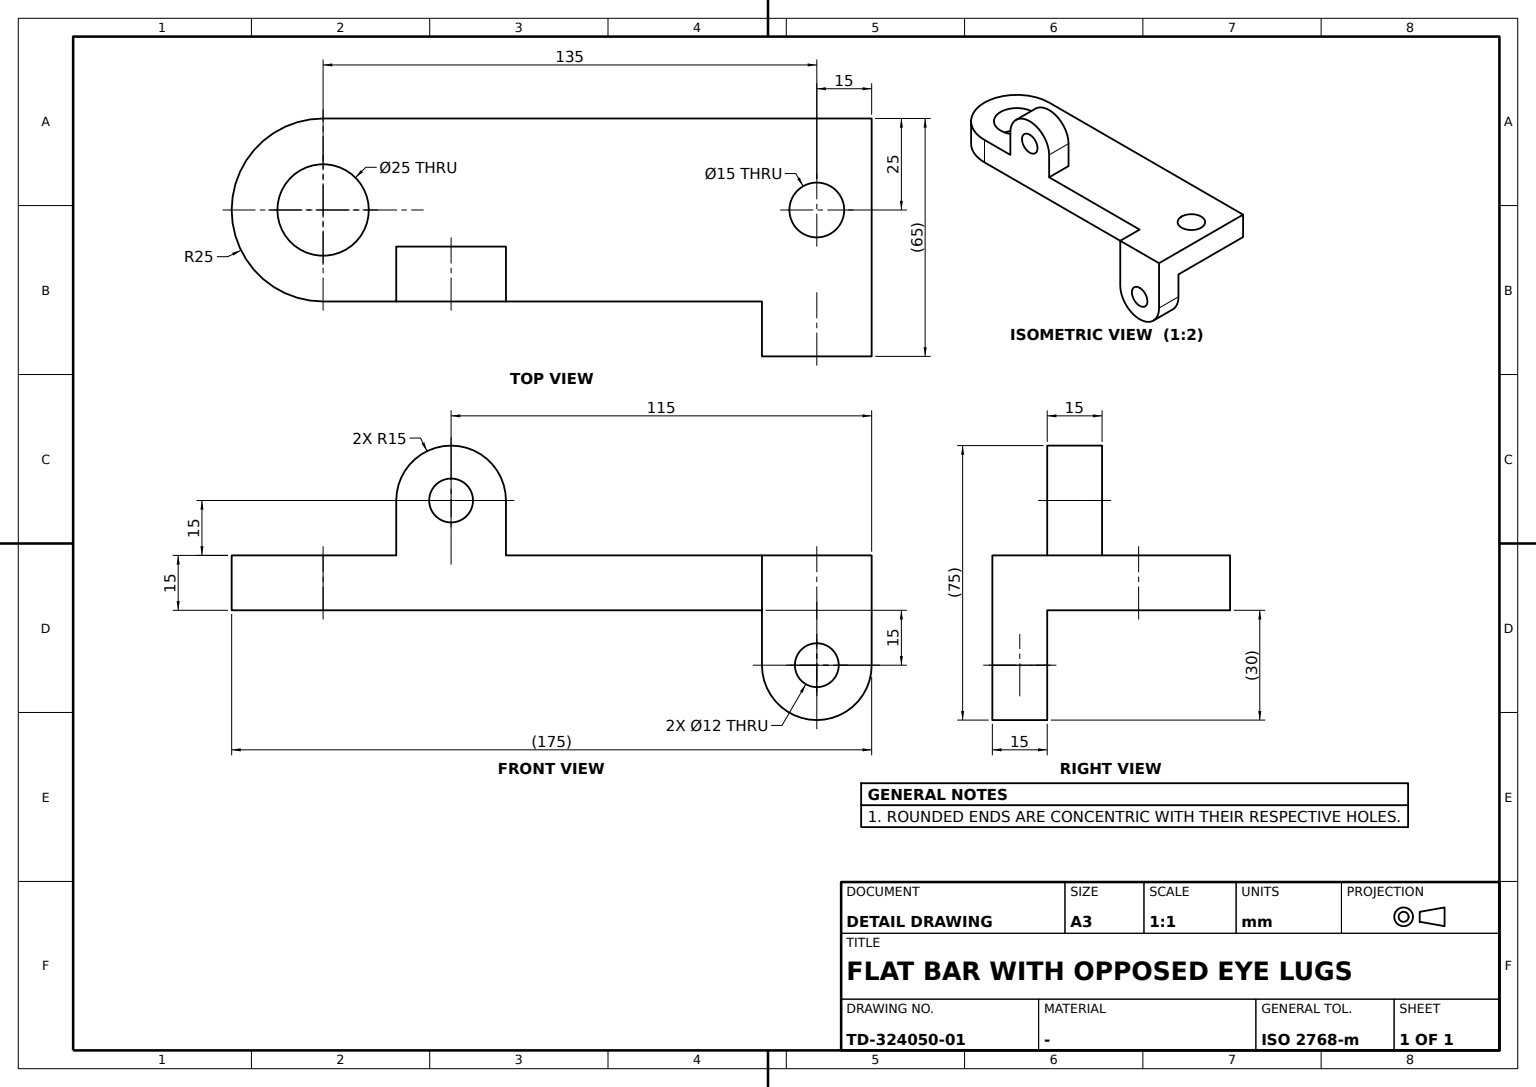
ISO-10303-21;
HEADER;
FILE_DESCRIPTION((''),'2;1');
FILE_NAME('','',(''),(''),'','','');
FILE_SCHEMA(('AUTOMOTIVE_DESIGN'));
ENDSEC;
DATA;
#1=APPLICATION_CONTEXT('');
#2=PRODUCT_CONTEXT('',#1,'mechanical');
#3=PRODUCT('','','',(#2));
#4=PRODUCT_DEFINITION_FORMATION('','',#3);
#5=PRODUCT_DEFINITION_CONTEXT('',#1,'design');
#6=PRODUCT_DEFINITION('','',#4,#5);
#7=PRODUCT_DEFINITION_SHAPE('','',#6);
#8=(LENGTH_UNIT()NAMED_UNIT(*)SI_UNIT(.MILLI.,.METRE.));
#9=(NAMED_UNIT(*)PLANE_ANGLE_UNIT()SI_UNIT($,.RADIAN.));
#10=(NAMED_UNIT(*)SI_UNIT($,.STERADIAN.)SOLID_ANGLE_UNIT());
#11=UNCERTAINTY_MEASURE_WITH_UNIT(LENGTH_MEASURE(0.005),#8,'distance_accuracy_value','');
#12=(GEOMETRIC_REPRESENTATION_CONTEXT(3)GLOBAL_UNCERTAINTY_ASSIGNED_CONTEXT((#11))GLOBAL_UNIT_ASSIGNED_CONTEXT((#8,#9,#10))REPRESENTATION_CONTEXT('',''));
#13=CARTESIAN_POINT('',(127.5,0.,-15.));
#14=VERTEX_POINT('',#13);
#15=CARTESIAN_POINT('',(127.5,0.,0.));
#16=VERTEX_POINT('',#15);
#17=DIRECTION('',(0.,0.,-1.));
#18=VECTOR('',#17,1000.);
#19=LINE('',#15,#18);
#20=EDGE_CURVE('',#14,#16,#19,.F.);
#21=ORIENTED_EDGE('',*,*,#20,.F.);
#22=CARTESIAN_POINT('',(142.5,0.,-15.));
#23=VERTEX_POINT('',#22);
#24=CARTESIAN_POINT('',(135.,0.,-15.));
#25=DIRECTION('',(0.,0.,1.));
#26=DIRECTION('',(1.,0.,0.));
#27=AXIS2_PLACEMENT_3D('',#24,#25,#26);
#28=CIRCLE('',#27,7.5);
#29=EDGE_CURVE('',#23,#14,#28,.T.);
#30=ORIENTED_EDGE('',*,*,#29,.F.);
#31=CARTESIAN_POINT('',(142.5,0.,0.));
#32=VERTEX_POINT('',#31);
#33=LINE('',#31,#18);
#34=EDGE_CURVE('',#32,#23,#33,.T.);
#35=ORIENTED_EDGE('',*,*,#34,.F.);
#36=CARTESIAN_POINT('',(135.,0.,0.));
#37=AXIS2_PLACEMENT_3D('',#36,#25,#26);
#38=CIRCLE('',#37,7.5);
#39=EDGE_CURVE('',#32,#16,#38,.T.);
#40=ORIENTED_EDGE('',*,*,#39,.T.);
#41=EDGE_LOOP('',(#21,#30,#35,#40));
#42=FACE_BOUND('',#41,.T.);
#43=DIRECTION('',(-1.,0.,0.));
#44=AXIS2_PLACEMENT_3D('',#36,#17,#43);
#45=CYLINDRICAL_SURFACE('',#44,7.5);
#46=ADVANCED_FACE('',(#42),#45,.F.);
#47=CARTESIAN_POINT('',(35.,-25.,30.));
#48=VERTEX_POINT('',#47);
#49=CARTESIAN_POINT('',(35.,-10.,30.));
#50=VERTEX_POINT('',#49);
#51=DIRECTION('',(0.,1.,0.));
#52=VECTOR('',#51,1000.);
#53=LINE('',#47,#52);
#54=EDGE_CURVE('',#48,#50,#53,.T.);
#55=ORIENTED_EDGE('',*,*,#54,.T.);
#56=CARTESIAN_POINT('',(20.,-10.,15.));
#57=VERTEX_POINT('',#56);
#58=CARTESIAN_POINT('',(35.,-10.,15.));
#59=DIRECTION('',(0.,-1.,0.));
#60=AXIS2_PLACEMENT_3D('',#58,#59,#26);
#61=CIRCLE('',#60,15.);
#62=EDGE_CURVE('',#50,#57,#61,.T.);
#63=ORIENTED_EDGE('',*,*,#62,.T.);
#64=CARTESIAN_POINT('',(20.,-25.,15.));
#65=VERTEX_POINT('',#64);
#66=LINE('',#64,#52);
#67=EDGE_CURVE('',#65,#57,#66,.T.);
#68=ORIENTED_EDGE('',*,*,#67,.F.);
#69=CARTESIAN_POINT('',(35.,-25.,15.));
#70=AXIS2_PLACEMENT_3D('',#69,#59,#26);
#71=CIRCLE('',#70,15.);
#72=EDGE_CURVE('',#48,#65,#71,.T.);
#73=ORIENTED_EDGE('',*,*,#72,.F.);
#74=EDGE_LOOP('',(#55,#63,#68,#73));
#75=FACE_BOUND('',#74,.T.);
#76=AXIS2_PLACEMENT_3D('',#69,#51,#25);
#77=CYLINDRICAL_SURFACE('',#76,15.);
#78=ADVANCED_FACE('',(#75),#77,.T.);
#79=CARTESIAN_POINT('',(50.,-25.,15.));
#80=VERTEX_POINT('',#79);
#81=EDGE_CURVE('',#80,#48,#71,.T.);
#82=ORIENTED_EDGE('',*,*,#81,.F.);
#83=CARTESIAN_POINT('',(50.,-10.,15.));
#84=VERTEX_POINT('',#83);
#85=LINE('',#79,#52);
#86=EDGE_CURVE('',#80,#84,#85,.T.);
#87=ORIENTED_EDGE('',*,*,#86,.T.);
#88=EDGE_CURVE('',#84,#50,#61,.T.);
#89=ORIENTED_EDGE('',*,*,#88,.T.);
#90=ORIENTED_EDGE('',*,*,#54,.F.);
#91=EDGE_LOOP('',(#82,#87,#89,#90));
#92=FACE_BOUND('',#91,.T.);
#93=ADVANCED_FACE('',(#92),#77,.T.);
#94=CARTESIAN_POINT('',(135.,-25.,-36.));
#95=VERTEX_POINT('',#94);
#96=CARTESIAN_POINT('',(135.,-25.,-24.));
#97=VERTEX_POINT('',#96);
#98=CARTESIAN_POINT('',(135.,-25.,-30.));
#99=AXIS2_PLACEMENT_3D('',#98,#59,#26);
#100=CIRCLE('',#99,6.);
#101=EDGE_CURVE('',#95,#97,#100,.T.);
#102=ORIENTED_EDGE('',*,*,#101,.T.);
#103=EDGE_CURVE('',#97,#95,#100,.T.);
#104=ORIENTED_EDGE('',*,*,#103,.T.);
#105=EDGE_LOOP('',(#102,#104));
#106=FACE_BOUND('',#105,.T.);
#107=CARTESIAN_POINT('',(120.,-25.,-15.));
#108=VERTEX_POINT('',#107);
#109=CARTESIAN_POINT('',(150.,-25.,-15.));
#110=VERTEX_POINT('',#109);
#111=CARTESIAN_POINT('',(0.,-25.,-15.));
#112=VECTOR('',#26,1000.);
#113=LINE('',#111,#112);
#114=EDGE_CURVE('',#108,#110,#113,.T.);
#115=ORIENTED_EDGE('',*,*,#114,.T.);
#116=CARTESIAN_POINT('',(150.,-25.,-30.));
#117=VERTEX_POINT('',#116);
#118=VECTOR('',#25,1000.);
#119=LINE('',#116,#118);
#120=EDGE_CURVE('',#117,#110,#119,.T.);
#121=ORIENTED_EDGE('',*,*,#120,.F.);
#122=CARTESIAN_POINT('',(135.,-25.,-45.));
#123=VERTEX_POINT('',#122);
#124=CIRCLE('',#99,15.);
#125=EDGE_CURVE('',#123,#117,#124,.T.);
#126=ORIENTED_EDGE('',*,*,#125,.F.);
#127=CARTESIAN_POINT('',(120.,-25.,-30.));
#128=VERTEX_POINT('',#127);
#129=EDGE_CURVE('',#128,#123,#124,.T.);
#130=ORIENTED_EDGE('',*,*,#129,.F.);
#131=CARTESIAN_POINT('',(120.,-25.,0.));
#132=LINE('',#131,#18);
#133=EDGE_CURVE('',#108,#128,#132,.T.);
#134=ORIENTED_EDGE('',*,*,#133,.F.);
#135=EDGE_LOOP('',(#115,#121,#126,#130,#134));
#136=FACE_BOUND('',#135,.T.);
#137=AXIS2_PLACEMENT_3D('',#98,#59,#17);
#138=PLANE('',#137);
#139=ADVANCED_FACE('',(#106,#136),#138,.F.);
#140=CARTESIAN_POINT('',(135.,-40.,-24.));
#141=VERTEX_POINT('',#140);
#142=VECTOR('',#59,1000.);
#143=LINE('',#96,#142);
#144=EDGE_CURVE('',#141,#97,#143,.F.);
#145=ORIENTED_EDGE('',*,*,#144,.T.);
#146=ORIENTED_EDGE('',*,*,#101,.F.);
#147=CARTESIAN_POINT('',(135.,-40.,-36.));
#148=VERTEX_POINT('',#147);
#149=LINE('',#94,#142);
#150=EDGE_CURVE('',#95,#148,#149,.T.);
#151=ORIENTED_EDGE('',*,*,#150,.T.);
#152=CARTESIAN_POINT('',(135.,-40.,-30.));
#153=AXIS2_PLACEMENT_3D('',#152,#59,#26);
#154=CIRCLE('',#153,6.);
#155=EDGE_CURVE('',#148,#141,#154,.T.);
#156=ORIENTED_EDGE('',*,*,#155,.T.);
#157=EDGE_LOOP('',(#145,#146,#151,#156));
#158=FACE_BOUND('',#157,.T.);
#159=CYLINDRICAL_SURFACE('',#137,6.);
#160=ADVANCED_FACE('',(#158),#159,.F.);
#161=ORIENTED_EDGE('',*,*,#86,.F.);
#162=CARTESIAN_POINT('',(50.,-25.,0.));
#163=VERTEX_POINT('',#162);
#164=LINE('',#162,#118);
#165=EDGE_CURVE('',#163,#80,#164,.T.);
#166=ORIENTED_EDGE('',*,*,#165,.F.);
#167=CARTESIAN_POINT('',(50.,-10.,0.));
#168=VERTEX_POINT('',#167);
#169=LINE('',#162,#52);
#170=EDGE_CURVE('',#163,#168,#169,.T.);
#171=ORIENTED_EDGE('',*,*,#170,.T.);
#172=LINE('',#167,#118);
#173=EDGE_CURVE('',#168,#84,#172,.T.);
#174=ORIENTED_EDGE('',*,*,#173,.T.);
#175=EDGE_LOOP('',(#161,#166,#171,#174));
#176=FACE_BOUND('',#175,.T.);
#177=AXIS2_PLACEMENT_3D('',#162,#43,#25);
#178=PLANE('',#177);
#179=ADVANCED_FACE('',(#176),#178,.F.);
#180=EDGE_CURVE('',#16,#32,#38,.T.);
#181=ORIENTED_EDGE('',*,*,#180,.T.);
#182=ORIENTED_EDGE('',*,*,#34,.T.);
#183=EDGE_CURVE('',#14,#23,#28,.T.);
#184=ORIENTED_EDGE('',*,*,#183,.F.);
#185=ORIENTED_EDGE('',*,*,#20,.T.);
#186=EDGE_LOOP('',(#181,#182,#184,#185));
#187=FACE_BOUND('',#186,.T.);
#188=ADVANCED_FACE('',(#187),#45,.F.);
#189=CARTESIAN_POINT('',(150.,25.,-15.));
#190=VERTEX_POINT('',#189);
#191=LINE('',#109,#52);
#192=EDGE_CURVE('',#110,#190,#191,.T.);
#193=ORIENTED_EDGE('',*,*,#192,.T.);
#194=CARTESIAN_POINT('',(150.,25.,0.));
#195=VERTEX_POINT('',#194);
#196=LINE('',#194,#18);
#197=EDGE_CURVE('',#195,#190,#196,.T.);
#198=ORIENTED_EDGE('',*,*,#197,.F.);
#199=CARTESIAN_POINT('',(150.,-40.,0.));
#200=VERTEX_POINT('',#199);
#201=CARTESIAN_POINT('',(150.,-25.,0.));
#202=LINE('',#201,#52);
#203=EDGE_CURVE('',#200,#195,#202,.T.);
#204=ORIENTED_EDGE('',*,*,#203,.F.);
#205=CARTESIAN_POINT('',(150.,-40.,-30.));
#206=VERTEX_POINT('',#205);
#207=LINE('',#205,#118);
#208=EDGE_CURVE('',#206,#200,#207,.T.);
#209=ORIENTED_EDGE('',*,*,#208,.F.);
#210=LINE('',#116,#142);
#211=EDGE_CURVE('',#117,#206,#210,.T.);
#212=ORIENTED_EDGE('',*,*,#211,.F.);
#213=ORIENTED_EDGE('',*,*,#120,.T.);
#214=EDGE_LOOP('',(#193,#198,#204,#209,#212,#213));
#215=FACE_BOUND('',#214,.T.);
#216=AXIS2_PLACEMENT_3D('',#201,#43,#25);
#217=PLANE('',#216);
#218=ADVANCED_FACE('',(#215),#217,.F.);
#219=CARTESIAN_POINT('',(-25.,0.,-15.));
#220=VERTEX_POINT('',#219);
#221=VERTEX_POINT('',#111);
#222=CARTESIAN_POINT('',(0.,0.,-15.));
#223=AXIS2_PLACEMENT_3D('',#222,#25,#26);
#224=CIRCLE('',#223,25.);
#225=EDGE_CURVE('',#220,#221,#224,.T.);
#226=ORIENTED_EDGE('',*,*,#225,.T.);
#227=CARTESIAN_POINT('',(0.,-25.,0.));
#228=VERTEX_POINT('',#227);
#229=LINE('',#227,#18);
#230=EDGE_CURVE('',#228,#221,#229,.T.);
#231=ORIENTED_EDGE('',*,*,#230,.F.);
#232=CARTESIAN_POINT('',(-25.,0.,0.));
#233=VERTEX_POINT('',#232);
#234=CARTESIAN_POINT('',(0.,0.,0.));
#235=AXIS2_PLACEMENT_3D('',#234,#25,#26);
#236=CIRCLE('',#235,25.);
#237=EDGE_CURVE('',#233,#228,#236,.T.);
#238=ORIENTED_EDGE('',*,*,#237,.F.);
#239=LINE('',#232,#18);
#240=EDGE_CURVE('',#233,#220,#239,.T.);
#241=ORIENTED_EDGE('',*,*,#240,.T.);
#242=EDGE_LOOP('',(#226,#231,#238,#241));
#243=FACE_BOUND('',#242,.T.);
#244=AXIS2_PLACEMENT_3D('',#234,#17,#43);
#245=CYLINDRICAL_SURFACE('',#244,25.);
#246=ADVANCED_FACE('',(#243),#245,.T.);
#247=EDGE_CURVE('',#221,#108,#113,.T.);
#248=ORIENTED_EDGE('',*,*,#247,.T.);
#249=VERTEX_POINT('',#131);
#250=EDGE_CURVE('',#249,#108,#132,.T.);
#251=ORIENTED_EDGE('',*,*,#250,.F.);
#252=LINE('',#227,#112);
#253=EDGE_CURVE('',#163,#249,#252,.T.);
#254=ORIENTED_EDGE('',*,*,#253,.F.);
#255=ORIENTED_EDGE('',*,*,#165,.T.);
#256=ORIENTED_EDGE('',*,*,#81,.T.);
#257=ORIENTED_EDGE('',*,*,#72,.T.);
#258=CARTESIAN_POINT('',(20.,-25.,0.));
#259=VERTEX_POINT('',#258);
#260=LINE('',#64,#18);
#261=EDGE_CURVE('',#65,#259,#260,.T.);
#262=ORIENTED_EDGE('',*,*,#261,.T.);
#263=EDGE_CURVE('',#228,#259,#252,.T.);
#264=ORIENTED_EDGE('',*,*,#263,.F.);
#265=ORIENTED_EDGE('',*,*,#230,.T.);
#266=EDGE_LOOP('',(#248,#251,#254,#255,#256,#257,#262,#264,#265));
#267=FACE_BOUND('',#266,.T.);
#268=CARTESIAN_POINT('',(35.,-25.,9.));
#269=VERTEX_POINT('',#268);
#270=CARTESIAN_POINT('',(35.,-25.,21.));
#271=VERTEX_POINT('',#270);
#272=CIRCLE('',#70,6.);
#273=EDGE_CURVE('',#269,#271,#272,.T.);
#274=ORIENTED_EDGE('',*,*,#273,.F.);
#275=EDGE_CURVE('',#271,#269,#272,.T.);
#276=ORIENTED_EDGE('',*,*,#275,.F.);
#277=EDGE_LOOP('',(#274,#276));
#278=FACE_BOUND('',#277,.T.);
#279=AXIS2_PLACEMENT_3D('',#227,#51,#25);
#280=PLANE('',#279);
#281=ADVANCED_FACE('',(#267,#278),#280,.F.);
#282=CARTESIAN_POINT('',(20.,-10.,0.));
#283=VERTEX_POINT('',#282);
#284=LINE('',#56,#18);
#285=EDGE_CURVE('',#57,#283,#284,.T.);
#286=ORIENTED_EDGE('',*,*,#285,.T.);
#287=LINE('',#258,#52);
#288=EDGE_CURVE('',#259,#283,#287,.T.);
#289=ORIENTED_EDGE('',*,*,#288,.F.);
#290=ORIENTED_EDGE('',*,*,#261,.F.);
#291=ORIENTED_EDGE('',*,*,#67,.T.);
#292=EDGE_LOOP('',(#286,#289,#290,#291));
#293=FACE_BOUND('',#292,.T.);
#294=AXIS2_PLACEMENT_3D('',#64,#26,#17);
#295=PLANE('',#294);
#296=ADVANCED_FACE('',(#293),#295,.F.);
#297=ORIENTED_EDGE('',*,*,#125,.T.);
#298=ORIENTED_EDGE('',*,*,#211,.T.);
#299=CARTESIAN_POINT('',(135.,-40.,-45.));
#300=VERTEX_POINT('',#299);
#301=CIRCLE('',#153,15.);
#302=EDGE_CURVE('',#300,#206,#301,.T.);
#303=ORIENTED_EDGE('',*,*,#302,.F.);
#304=LINE('',#122,#142);
#305=EDGE_CURVE('',#123,#300,#304,.T.);
#306=ORIENTED_EDGE('',*,*,#305,.F.);
#307=EDGE_LOOP('',(#297,#298,#303,#306));
#308=FACE_BOUND('',#307,.T.);
#309=CYLINDRICAL_SURFACE('',#137,15.);
#310=ADVANCED_FACE('',(#308),#309,.T.);
#311=CARTESIAN_POINT('',(-12.5,0.,0.));
#312=VERTEX_POINT('',#311);
#313=CARTESIAN_POINT('',(12.5,0.,0.));
#314=VERTEX_POINT('',#313);
#315=CIRCLE('',#235,12.5);
#316=EDGE_CURVE('',#312,#314,#315,.T.);
#317=ORIENTED_EDGE('',*,*,#316,.T.);
#318=CARTESIAN_POINT('',(12.5,0.,-15.));
#319=VERTEX_POINT('',#318);
#320=LINE('',#313,#18);
#321=EDGE_CURVE('',#314,#319,#320,.T.);
#322=ORIENTED_EDGE('',*,*,#321,.T.);
#323=CARTESIAN_POINT('',(-12.5,0.,-15.));
#324=VERTEX_POINT('',#323);
#325=CIRCLE('',#223,12.5);
#326=EDGE_CURVE('',#324,#319,#325,.T.);
#327=ORIENTED_EDGE('',*,*,#326,.F.);
#328=LINE('',#311,#18);
#329=EDGE_CURVE('',#324,#312,#328,.F.);
#330=ORIENTED_EDGE('',*,*,#329,.T.);
#331=EDGE_LOOP('',(#317,#322,#327,#330));
#332=FACE_BOUND('',#331,.T.);
#333=CYLINDRICAL_SURFACE('',#244,12.5);
#334=ADVANCED_FACE('',(#332),#333,.F.);
#335=EDGE_CURVE('',#319,#324,#325,.T.);
#336=ORIENTED_EDGE('',*,*,#335,.F.);
#337=ORIENTED_EDGE('',*,*,#321,.F.);
#338=EDGE_CURVE('',#314,#312,#315,.T.);
#339=ORIENTED_EDGE('',*,*,#338,.T.);
#340=ORIENTED_EDGE('',*,*,#329,.F.);
#341=EDGE_LOOP('',(#336,#337,#339,#340));
#342=FACE_BOUND('',#341,.T.);
#343=ADVANCED_FACE('',(#342),#333,.F.);
#344=ORIENTED_EDGE('',*,*,#39,.F.);
#345=ORIENTED_EDGE('',*,*,#180,.F.);
#346=EDGE_LOOP('',(#344,#345));
#347=FACE_BOUND('',#346,.T.);
#348=ORIENTED_EDGE('',*,*,#316,.F.);
#349=ORIENTED_EDGE('',*,*,#338,.F.);
#350=EDGE_LOOP('',(#348,#349));
#351=FACE_BOUND('',#350,.T.);
#352=CARTESIAN_POINT('',(0.,25.,0.));
#353=VERTEX_POINT('',#352);
#354=VECTOR('',#43,1000.);
#355=LINE('',#194,#354);
#356=EDGE_CURVE('',#195,#353,#355,.T.);
#357=ORIENTED_EDGE('',*,*,#356,.T.);
#358=EDGE_CURVE('',#353,#233,#236,.T.);
#359=ORIENTED_EDGE('',*,*,#358,.T.);
#360=ORIENTED_EDGE('',*,*,#237,.T.);
#361=ORIENTED_EDGE('',*,*,#263,.T.);
#362=ORIENTED_EDGE('',*,*,#288,.T.);
#363=LINE('',#282,#112);
#364=EDGE_CURVE('',#283,#168,#363,.T.);
#365=ORIENTED_EDGE('',*,*,#364,.T.);
#366=ORIENTED_EDGE('',*,*,#170,.F.);
#367=ORIENTED_EDGE('',*,*,#253,.T.);
#368=CARTESIAN_POINT('',(120.,-40.,0.));
#369=VERTEX_POINT('',#368);
#370=LINE('',#131,#142);
#371=EDGE_CURVE('',#249,#369,#370,.T.);
#372=ORIENTED_EDGE('',*,*,#371,.T.);
#373=LINE('',#199,#354);
#374=EDGE_CURVE('',#200,#369,#373,.T.);
#375=ORIENTED_EDGE('',*,*,#374,.F.);
#376=ORIENTED_EDGE('',*,*,#203,.T.);
#377=EDGE_LOOP('',(#357,#359,#360,#361,#362,#365,#366,#367,#372,#375,#376));
#378=FACE_BOUND('',#377,.T.);
#379=PLANE('',#235);
#380=ADVANCED_FACE('',(#347,#351,#378),#379,.T.);
#381=CARTESIAN_POINT('',(0.,25.,-15.));
#382=VERTEX_POINT('',#381);
#383=LINE('',#189,#354);
#384=EDGE_CURVE('',#190,#382,#383,.T.);
#385=ORIENTED_EDGE('',*,*,#384,.T.);
#386=LINE('',#352,#18);
#387=EDGE_CURVE('',#353,#382,#386,.T.);
#388=ORIENTED_EDGE('',*,*,#387,.F.);
#389=ORIENTED_EDGE('',*,*,#356,.F.);
#390=ORIENTED_EDGE('',*,*,#197,.T.);
#391=EDGE_LOOP('',(#385,#388,#389,#390));
#392=FACE_BOUND('',#391,.T.);
#393=AXIS2_PLACEMENT_3D('',#194,#59,#17);
#394=PLANE('',#393);
#395=ADVANCED_FACE('',(#392),#394,.F.);
#396=CARTESIAN_POINT('',(120.,-40.,-30.));
#397=VERTEX_POINT('',#396);
#398=EDGE_CURVE('',#397,#300,#301,.T.);
#399=ORIENTED_EDGE('',*,*,#398,.F.);
#400=LINE('',#127,#142);
#401=EDGE_CURVE('',#128,#397,#400,.T.);
#402=ORIENTED_EDGE('',*,*,#401,.F.);
#403=ORIENTED_EDGE('',*,*,#129,.T.);
#404=ORIENTED_EDGE('',*,*,#305,.T.);
#405=EDGE_LOOP('',(#399,#402,#403,#404));
#406=FACE_BOUND('',#405,.T.);
#407=ADVANCED_FACE('',(#406),#309,.T.);
#408=CARTESIAN_POINT('',(35.,-10.,9.));
#409=VERTEX_POINT('',#408);
#410=LINE('',#268,#52);
#411=EDGE_CURVE('',#409,#269,#410,.F.);
#412=ORIENTED_EDGE('',*,*,#411,.T.);
#413=ORIENTED_EDGE('',*,*,#273,.T.);
#414=CARTESIAN_POINT('',(35.,-10.,21.));
#415=VERTEX_POINT('',#414);
#416=LINE('',#270,#52);
#417=EDGE_CURVE('',#271,#415,#416,.T.);
#418=ORIENTED_EDGE('',*,*,#417,.T.);
#419=CIRCLE('',#60,6.);
#420=EDGE_CURVE('',#409,#415,#419,.T.);
#421=ORIENTED_EDGE('',*,*,#420,.F.);
#422=EDGE_LOOP('',(#412,#413,#418,#421));
#423=FACE_BOUND('',#422,.T.);
#424=CYLINDRICAL_SURFACE('',#76,6.);
#425=ADVANCED_FACE('',(#423),#424,.F.);
#426=ORIENTED_EDGE('',*,*,#62,.F.);
#427=ORIENTED_EDGE('',*,*,#88,.F.);
#428=ORIENTED_EDGE('',*,*,#173,.F.);
#429=ORIENTED_EDGE('',*,*,#364,.F.);
#430=ORIENTED_EDGE('',*,*,#285,.F.);
#431=EDGE_LOOP('',(#426,#427,#428,#429,#430));
#432=FACE_BOUND('',#431,.T.);
#433=ORIENTED_EDGE('',*,*,#420,.T.);
#434=EDGE_CURVE('',#415,#409,#419,.T.);
#435=ORIENTED_EDGE('',*,*,#434,.T.);
#436=EDGE_LOOP('',(#433,#435));
#437=FACE_BOUND('',#436,.T.);
#438=AXIS2_PLACEMENT_3D('',#58,#59,#17);
#439=PLANE('',#438);
#440=ADVANCED_FACE('',(#432,#437),#439,.F.);
#441=LINE('',#368,#18);
#442=EDGE_CURVE('',#369,#397,#441,.T.);
#443=ORIENTED_EDGE('',*,*,#442,.T.);
#444=ORIENTED_EDGE('',*,*,#398,.T.);
#445=ORIENTED_EDGE('',*,*,#302,.T.);
#446=ORIENTED_EDGE('',*,*,#208,.T.);
#447=ORIENTED_EDGE('',*,*,#374,.T.);
#448=EDGE_LOOP('',(#443,#444,#445,#446,#447));
#449=FACE_BOUND('',#448,.T.);
#450=EDGE_CURVE('',#141,#148,#154,.T.);
#451=ORIENTED_EDGE('',*,*,#450,.F.);
#452=ORIENTED_EDGE('',*,*,#155,.F.);
#453=EDGE_LOOP('',(#451,#452));
#454=FACE_BOUND('',#453,.T.);
#455=AXIS2_PLACEMENT_3D('',#152,#59,#17);
#456=PLANE('',#455);
#457=ADVANCED_FACE('',(#449,#454),#456,.T.);
#458=ORIENTED_EDGE('',*,*,#417,.F.);
#459=ORIENTED_EDGE('',*,*,#275,.T.);
#460=ORIENTED_EDGE('',*,*,#411,.F.);
#461=ORIENTED_EDGE('',*,*,#434,.F.);
#462=EDGE_LOOP('',(#458,#459,#460,#461));
#463=FACE_BOUND('',#462,.T.);
#464=ADVANCED_FACE('',(#463),#424,.F.);
#465=ORIENTED_EDGE('',*,*,#450,.T.);
#466=ORIENTED_EDGE('',*,*,#150,.F.);
#467=ORIENTED_EDGE('',*,*,#103,.F.);
#468=ORIENTED_EDGE('',*,*,#144,.F.);
#469=EDGE_LOOP('',(#465,#466,#467,#468));
#470=FACE_BOUND('',#469,.T.);
#471=ADVANCED_FACE('',(#470),#159,.F.);
#472=ORIENTED_EDGE('',*,*,#358,.F.);
#473=ORIENTED_EDGE('',*,*,#387,.T.);
#474=EDGE_CURVE('',#382,#220,#224,.T.);
#475=ORIENTED_EDGE('',*,*,#474,.T.);
#476=ORIENTED_EDGE('',*,*,#240,.F.);
#477=EDGE_LOOP('',(#472,#473,#475,#476));
#478=FACE_BOUND('',#477,.T.);
#479=ADVANCED_FACE('',(#478),#245,.T.);
#480=ORIENTED_EDGE('',*,*,#250,.T.);
#481=ORIENTED_EDGE('',*,*,#133,.T.);
#482=ORIENTED_EDGE('',*,*,#401,.T.);
#483=ORIENTED_EDGE('',*,*,#442,.F.);
#484=ORIENTED_EDGE('',*,*,#371,.F.);
#485=EDGE_LOOP('',(#480,#481,#482,#483,#484));
#486=FACE_BOUND('',#485,.T.);
#487=AXIS2_PLACEMENT_3D('',#131,#43,#25);
#488=PLANE('',#487);
#489=ADVANCED_FACE('',(#486),#488,.T.);
#490=ORIENTED_EDGE('',*,*,#326,.T.);
#491=ORIENTED_EDGE('',*,*,#335,.T.);
#492=EDGE_LOOP('',(#490,#491));
#493=FACE_BOUND('',#492,.T.);
#494=ORIENTED_EDGE('',*,*,#114,.F.);
#495=ORIENTED_EDGE('',*,*,#247,.F.);
#496=ORIENTED_EDGE('',*,*,#225,.F.);
#497=ORIENTED_EDGE('',*,*,#474,.F.);
#498=ORIENTED_EDGE('',*,*,#384,.F.);
#499=ORIENTED_EDGE('',*,*,#192,.F.);
#500=EDGE_LOOP('',(#494,#495,#496,#497,#498,#499));
#501=FACE_BOUND('',#500,.T.);
#502=ORIENTED_EDGE('',*,*,#29,.T.);
#503=ORIENTED_EDGE('',*,*,#183,.T.);
#504=EDGE_LOOP('',(#502,#503));
#505=FACE_BOUND('',#504,.T.);
#506=PLANE('',#223);
#507=ADVANCED_FACE('',(#493,#501,#505),#506,.F.);
#508=CLOSED_SHELL('',(#46,#78,#93,#139,#160,#179,#188,#218,#246,#281,#296,#310,#334,#343,#380,#395,#407,#425,#440,#457,#464,#471,#479,#489,#507));
#509=MANIFOLD_SOLID_BREP('',#508);
#510=ADVANCED_BREP_SHAPE_REPRESENTATION('',(#509),#12);
#511=SHAPE_DEFINITION_REPRESENTATION(#7,#510);
ENDSEC;
END-ISO-10303-21;
